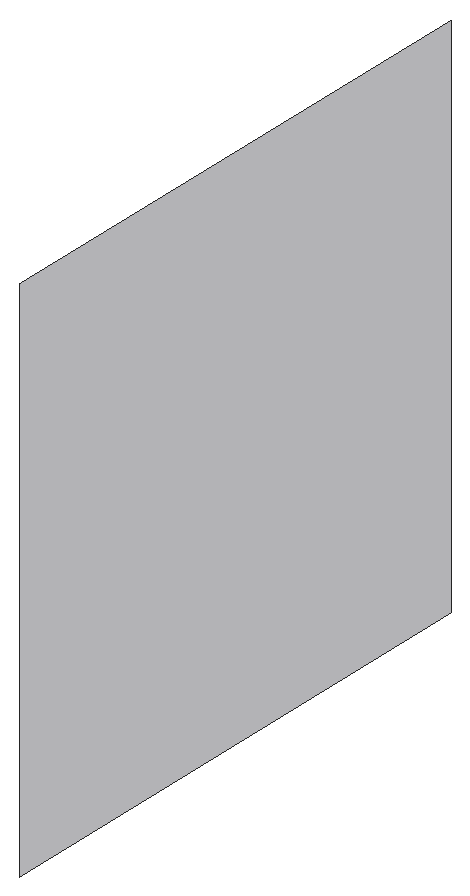
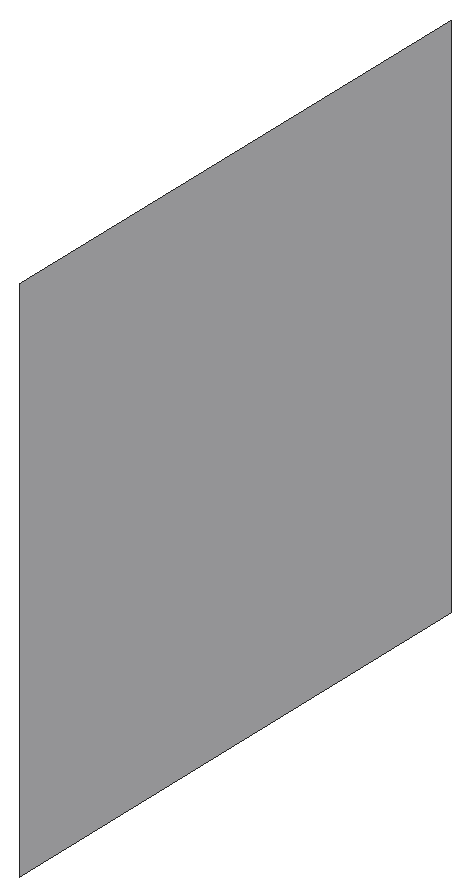
# SketchUp Ruby script. Lengths in inches.
U = 1.inch
M = Sketchup.active_model
def pt(a) = Geom::Point3d.new(a.map { |v| v * U })
def face(e, loops, mat)
  f = e.add_face(loops[0].map { |a| pt(a) })
  loops[1..].each { |l| e.add_face(l.map { |a| pt(a) }).erase! }
  f.material = f.back_material = mat if mat
  f
end
# faces: each face lists its corners as indices into pts; further lists are holes
def faces(e, pts, list, mat = nil) = list.each { |f| face(e, (f[0].is_a?(Array) ? f : [f]).map { |l| l.map { |i| pts[i] } }, mat) }
# xy, xz, yz: faces in a plane at the given z, y or x. An outline is a flat list of corners, or four numbers for a rectangle; further outlines are holes
def ring(l) = l.size == 4 ? [[l[0], l[1]], [l[2], l[1]], [l[2], l[3]], [l[0], l[3]]] : l.each_slice(2).to_a
def flat(e, list, mat, &to3) = list.each { |f| face(e, (f[0].is_a?(Array) ? f : [f]).map { |l| ring(l).map { |u, v| to3.(u, v) } }, mat) }
def xy(e, z, list, mat = nil) = flat(e, list, mat) { |x, y| [x, y, z] }
def xz(e, y, list, mat = nil) = flat(e, list, mat) { |x, z| [x, y, z] }
def yz(e, x, list, mat = nil) = flat(e, list, mat) { |y, z| [x, y, z] }
def lines(e, pts, list) = list.each { |a, b| e.add_line(pt(pts[a]), pt(pts[b])) }
# prism: a flat outline (further loops are holes) pulled along v
def prism(e, loops, v, mat = nil)
  f = face(e, loops, mat); d = Geom::Vector3d.new(v.map { |x| x * U })
  f.pushpull(f.normal.samedirection?(d) ? d.length : -d.length)
end
def box(e, o, s, mat = nil) = prism(e, [[o, [o[0] + s[0], o[1], o[2]], [o[0] + s[0], o[1] + s[1], o[2]], [o[0], o[1] + s[1], o[2]]]], [0, 0, s[2]], mat)
def at(x, y, z, deg = 0) = Geom::Transformation.translation(pt([x, y, z])) * Geom::Transformation.rotation(ORIGIN, Z_AXIS, deg.degrees)
def axes(o, x, y, z) = Geom::Transformation.new([*x, 0, *y, 0, *z, 0, *pt(o).to_a, 1])
def part(name) = M.definitions.add(name)
# library, detail: a bought-in or finely detailed component or shape, given as its bounding box
def library(name, o, s) = part(name).tap { |d| box(d.entities, o, s) }
def detail(e, o, s) = box(e.add_group.entities, o, s)
def put(e, d, t, mat = nil) = e.add_instance(d, t).tap { |i| i.material = mat if mat }
def group(e, t, mat = nil) = e.add_group.tap { |g| g.transformation = t; g.material = mat if mat }.entities
root = M.entities
M.materials.add("[Blinds Vertical Pattern]1").color = [239, 239, 242]
yz(root,213.78,[[96.24,37.78,111,52.34]],"[Blinds Vertical Pattern]1")
